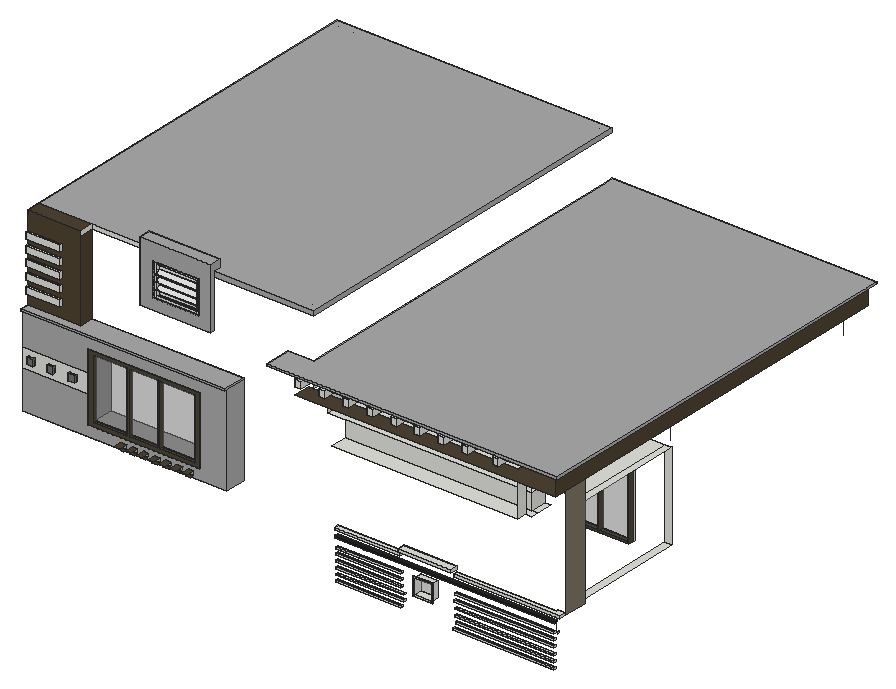
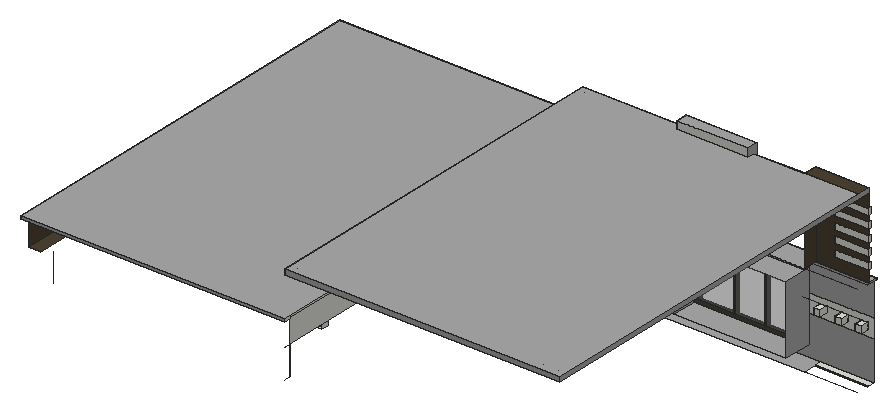
# SketchUp Ruby script. Lengths in inches.
U = 1.inch
M = Sketchup.active_model
def pt(a) = Geom::Point3d.new(a.map { |v| v * U })
def face(e, loops, mat)
  f = e.add_face(loops[0].map { |a| pt(a) })
  loops[1..].each { |l| e.add_face(l.map { |a| pt(a) }).erase! }
  f.material = f.back_material = mat if mat
  f
end
# faces: each face lists its corners as indices into pts; further lists are holes
def faces(e, pts, list, mat = nil) = list.each { |f| face(e, (f[0].is_a?(Array) ? f : [f]).map { |l| l.map { |i| pts[i] } }, mat) }
# xy, xz, yz: faces in a plane at the given z, y or x. An outline is a flat list of corners, or four numbers for a rectangle; further outlines are holes
def ring(l) = l.size == 4 ? [[l[0], l[1]], [l[2], l[1]], [l[2], l[3]], [l[0], l[3]]] : l.each_slice(2).to_a
def flat(e, list, mat, &to3) = list.each { |f| face(e, (f[0].is_a?(Array) ? f : [f]).map { |l| ring(l).map { |u, v| to3.(u, v) } }, mat) }
def xy(e, z, list, mat = nil) = flat(e, list, mat) { |x, y| [x, y, z] }
def xz(e, y, list, mat = nil) = flat(e, list, mat) { |x, z| [x, y, z] }
def yz(e, x, list, mat = nil) = flat(e, list, mat) { |y, z| [x, y, z] }
def lines(e, pts, list) = list.each { |a, b| e.add_line(pt(pts[a]), pt(pts[b])) }
# prism: a flat outline (further loops are holes) pulled along v
def prism(e, loops, v, mat = nil)
  f = face(e, loops, mat); d = Geom::Vector3d.new(v.map { |x| x * U })
  f.pushpull(f.normal.samedirection?(d) ? d.length : -d.length)
end
def box(e, o, s, mat = nil) = prism(e, [[o, [o[0] + s[0], o[1], o[2]], [o[0] + s[0], o[1] + s[1], o[2]], [o[0], o[1] + s[1], o[2]]]], [0, 0, s[2]], mat)
def at(x, y, z, deg = 0) = Geom::Transformation.translation(pt([x, y, z])) * Geom::Transformation.rotation(ORIGIN, Z_AXIS, deg.degrees)
def axes(o, x, y, z) = Geom::Transformation.new([*x, 0, *y, 0, *z, 0, *pt(o).to_a, 1])
def part(name) = M.definitions.add(name)
# library, detail: a bought-in or finely detailed component or shape, given as its bounding box
def library(name, o, s) = part(name).tap { |d| box(d.entities, o, s) }
def detail(e, o, s) = box(e.add_group.entities, o, s)
def put(e, d, t, mat = nil) = e.add_instance(d, t).tap { |i| i.material = mat if mat }
def group(e, t, mat = nil) = e.add_group.tap { |g| g.transformation = t; g.material = mat if mat }.entities
root = M.entities
M.materials.add("[Color B08]").color = [76, 71, 58]
M.materials.add("[Color C08]").color = [78, 67, 50]
M.materials.add("[Color M03]").color = [170, 170, 170]
M.materials.add("[Color M05]").color = [114, 114, 114]
M.materials.add("[Color M08]").color = [30, 30, 30]
M.materials.add("[Mirror 02]").color = [229, 229, 229]
M.materials.add("[Stone Flagstone Ashlar]1").color = [126, 116, 102]
M.materials.add("[Translucent Glass Gray]").color = [128, 128, 128]
M.materials["[Translucent Glass Gray]"].alpha = 0.5
c1 = part("Group\#2")
xy(c1.entities,0,[[0,0,90.375,3.1875]],"[Color B08]")
xy(c1.entities,4.18,[[4.18,0,31.5,3.1875],[31.5,0,33.18,3.1875],[33.18,0,56.375,3.1875],[56.375,0,58.06,3.1875],[58.06,0,86.19,3.1875]],"[Color B08]")
xy(c1.entities,71.26,[[4.18,0,31.5,3.1875],[33.18,0,56.375,3.1875],[58.06,0,86.19,3.1875]],"[Color B08]")
xy(c1.entities,75.4375,[[0,0,90.375,3.1875]],"[Color B08]")
xz(c1.entities,0,[[[0,0,90.375,75.4375],[4.18,4.18,4.18,71.26,31.5,71.26,31.5,4.18,33.18,4.18,33.18,71.26,56.375,71.26,56.375,4.18,58.06,4.18,58.06,71.26,86.19,71.26,86.19,4.18]]],"[Color B08]")
xz(c1.entities,3.1875,[[[0,0,90.375,75.4375],[4.18,4.18,86.19,4.18,86.19,71.26,58.06,71.26,58.06,4.18,56.375,4.18,56.375,71.26,33.18,71.26,33.18,4.18,31.5,4.18,31.5,71.26,4.18,71.26]]],"[Color B08]")
xz(c1.entities,3.1875,[[4.18,4.18,31.5,71.26],[33.18,4.18,56.375,71.26],[58.06,4.18,86.19,71.26]],"[Translucent Glass Gray]")
yz(c1.entities,0,[[0,0,3.1875,75.4375]],"[Color B08]")
yz(c1.entities,4.18,[[0,4.18,3.1875,71.26]],"[Color B08]")
yz(c1.entities,31.5,[[0,4.18,3.1875,71.26]],"[Color B08]")
yz(c1.entities,33.18,[[0,4.18,3.1875,71.26]],"[Color B08]")
yz(c1.entities,56.375,[[0,4.18,3.1875,71.26]],"[Color B08]")
yz(c1.entities,58.06,[[0,4.18,3.1875,71.26]],"[Color B08]")
yz(c1.entities,86.19,[[0,4.18,3.1875,71.26]],"[Color B08]")
yz(c1.entities,90.375,[[0,0,3.1875,75.4375]],"[Color B08]")
box(root,[394.1875,137.57,204.05],[82.8125,1.69,1.43])
box(root,[395.9375,137.57,209.3],[81.0625,1.69,1.43])
box(root,[297.76,137.5,210.54],[56,1.68,1.43])
box(root,[395.5625,137.57,214.55],[81.4375,1.69,1.43])
box(root,[297.76,137.5,215.47],[55.93,1.68,1.44])
box(root,[395.4375,137.57,219.8],[81.5625,1.69,1.43])
box(root,[395.0625,137.57,225.05],[81.9375,1.69,1.43])
xy(root,205.6,[[297.76,137.5,351.41,139.18]])
xy(root,207.04,[[297.76,137.5,351.41,139.18]])
xy(root,220.41,[[297.76,137.5,351.41,139.18]])
xy(root,220.77,[[364.68,133.4375,380.63,134]])
xy(root,221.65,[[365.56,133.4375,379.75,140]])
xy(root,221.85,[[297.76,137.5,351.41,139.18]])
xy(root,225.35,[[297.76,137.5,351.41,139.18]])
xy(root,226.79,[[297.76,137.5,351.41,139.18]])
xy(root,230.29,[[297.76,137.5,351.41,139.18]])
xy(root,230.3,[[395.45,137.57,477,139.26]])
xy(root,231.72,[[297.76,137.5,351.41,139.18]])
xy(root,231.73,[[395.45,137.57,477,139.26]])
xy(root,234.53,[[365.56,133.4375,379.75,140]])
xy(root,235.41,[[364.68,133.4375,380.63,134]])
xy(root,236.42,[[398.45,250.9375,448.01,256.9375]])
xy(root,238.64,[[321.84,136.1875,324.02,136.85],[436.79,136.1875,439.16,136.85],[297.76,136.85,321.84,139.48],[321.84,136.85,324.02,139.48],[324.02,136.85,436.79,139.48],
  [436.79,136.85,439.16,139.48],[439.16,136.85,477.88,139.48],[321.84,139.48,324.02,140],[436.79,139.48,439.16,140]],"[Color M08]")
xy(root,240.27,[[297.76,136.85,477.88,139.48]],"[Color M08]")
xy(root,244.375,[[297.76,136.1875,351.41,140],[395.45,136.1875,477,140],[477,136.1875,483,141.8125]])
xy(root,246.375,[[297.76,136.1875,351.41,140],[395.45,136.1875,483,136.1875,483,141.8125,477,141.8125,477,140,395.45,140]])
xy(root,248,[[351.41,134,395.45,140],[477,161.5,483,250.9375]])
xy(root,250.4375,[[351.41,134,395.45,140]])
xy(root,255.68,[[57,117.0625,100.7,122.5625],[57,122.5625,100.7,123.75]])
xy(root,255.68,[[100.7,117.0625,224.8125,134]],"[Color M03]")
xy(root,257.55,[[138.22,113.92,142.66,117.0625],[147.41,113.92,151.85,117.0625],[156.6,113.92,161.03,117.0625],[165.78,113.92,170.22,117.0625],[174.97,113.92,179.41,117.0625],
  [184.16,113.92,188.6,117.0625],[193.35,113.92,197.78,117.0625]],"[Color C08]")
xy(root,261.3,[[138.22,109.625,142.66,117.0625],[147.41,109.625,151.85,117.0625],[156.6,109.625,161.03,117.0625],[165.78,109.625,170.22,117.0625],[174.97,109.625,179.41,117.0625],
  [184.16,109.625,188.6,117.0625],[193.35,109.625,197.78,117.0625]],"[Color C08]")
xy(root,264.625,[[110.92,117.0625,202.92,140]],"[Color M03]")
xy(root,284,[[310.04,250.9375,358.04,256.9375]])
xy(root,291.17,[[398.45,250.9375,448.01,256.9375]])
xy(root,292.91,[[61.94,117.0625,67.26,123.75],[78.26,117.0625,83.57,123.75],[96.13,117.0625,101.44,123.75]])
xy(root,292.91,[[61.94,115.0625,67.26,117.0625],[78.26,115.0625,83.57,117.0625],[96.13,115.0625,101.44,117.0625]],"[Color M05]")
xy(root,298.22,[[61.94,117.0625,67.26,123.75],[78.26,117.0625,83.57,123.75],[96.13,117.0625,101.44,123.75]])
xy(root,298.22,[[61.94,115.0625,67.26,117.0625],[78.26,115.0625,83.57,117.0625],[96.13,115.0625,101.44,117.0625]],"[Color M05]")
xy(root,307.0625,[[297.76,134,297.76,148.25,455.38,148.25,455.38,141.8125,450.07,141.8125,450.07,134],[450.07,148.25,455.38,161.5]])
xy(root,320,[[282.75,148.25,282.75,250.9375,477,250.9375,477,161.5,450.07,161.5,450.07,148.25],[477,161.5,483,250.9375]])
xy(root,320.75,[[110.92,117.0625,202.92,140]],"[Color M03]")
xy(root,330.3,[[57,114.8125,224.8125,117.0625]],"[Color M03]")
xy(root,331.68,[[57,114.8125,224.8125,114.8125,224.8125,134,100.7,134,100.7,122.5625,57,122.5625]],"[Color M03]")
xy(root,340.7,[[57,120.3125,85,122.5625]])
xy(root,344,[[278.5625,119.875,278.5625,134,450.07,134,450.07,141.8125,483,141.8125,483,440,492.4375,440,492.4375,119.875]],"[Color C08]")
xy(root,345.82,[[57,120.3125,85,122.5625]])
xy(root,350.76,[[57,120.3125,85,122.5625]])
xy(root,355.88,[[57,120.3125,85,122.5625]])
xy(root,356.93,[[286.08,110.5,290.89,119.875],[305.64,110.5,310.46,119.875],[325.21,110.5,330.02,119.875],[344.77,110.5,349.58,119.875],[364.33,110.5,369.14,119.875],
  [383.89,110.5,388.71,119.875],[403.46,110.5,408.27,119.875],[423.02,110.5,427.83,119.875],[447.96,110.5,452.77,119.875]])
xy(root,358,[[142.38,130.5,200.45,134]],"[Color M03]")
xy(root,360.82,[[57,120.3125,85,122.5625]])
xy(root,362.625,[[286.08,110.5,290.89,112.3125],[305.64,110.5,310.46,112.3125],[325.21,110.5,330.02,112.3125],[344.77,110.5,349.58,112.3125],[364.33,110.5,369.14,112.3125],
  [383.89,110.5,388.71,112.3125],[403.46,110.5,408.27,112.3125],[423.02,110.5,427.83,112.3125],[447.96,110.5,452.77,112.3125],[264.5625,119.875,264.5625,134,282.75,134,282.75,256.9375,283.22,434,282.75,434,282.75,440,492.4375,440,492.4375,119.875]])
xy(root,362.625,[[261.625,112.3125,261.625,134,264.5625,134,264.5625,119.875,286.08,119.875,286.08,112.3125],[290.89,112.3125,305.64,119.875],[310.46,112.3125,325.21,119.875],[330.02,112.3125,344.77,119.875],[349.58,112.3125,364.33,119.875],
  [369.14,112.3125,383.89,119.875],[388.71,112.3125,403.46,119.875],[408.27,112.3125,423.02,119.875],[427.83,112.3125,447.96,119.875],[452.77,112.3125,452.77,119.875,492.4375,119.875,492.4375,440,499.5625,440,499.5625,112.3125]],"[Color M03]")
xy(root,364.625,[[261.625,112.3125,499.5625,112.3125,499.5625,440,282.75,440,282.75,434,283.22,434,282.75,256.9375,282.75,134,261.625,134]],"[Color M03]")
xy(root,365.95,[[57,120.3125,85,122.5625]])
xy(root,367.19,[[153.29,130.5,191.16,140]],"[Color M03]")
xy(root,370.88,[[57,120.3125,85,122.5625]])
xy(root,376.01,[[57,120.3125,85,122.5625]])
xy(root,380.95,[[57,120.3125,85,122.5625]])
xy(root,386.07,[[57,120.3125,85,122.5625]])
xy(root,394.44,[[153.29,130.5,191.16,140]],"[Color M03]")
xy(root,401.5625,[[57,122.5625,100.7,134]],"[Color C08]")
xy(root,401.5625,[[57,134,142.38,134,142.38,140,200.45,140,200.45,134,282.75,134,282.75,440,57,440]],"[Color M03]")
xy(root,408.0625,[[142.38,130.5,200.45,140]],"[Color M03]")
xz(root,110.5,[[286.08,356.93,290.89,362.625],[305.64,356.93,310.46,362.625],[325.21,356.93,330.02,362.625],[344.77,356.93,349.58,362.625],[364.33,356.93,369.14,362.625],
  [383.89,356.93,388.71,362.625],[403.46,356.93,408.27,362.625],[423.02,356.93,427.83,362.625],[447.96,356.93,452.77,362.625]])
xz(root,112.3125,[[261.625,362.625,499.5625,364.625]],"[Color M03]")
xz(root,114.8125,[[57,330.3,224.8125,331.68]],"[Color M03]")
xz(root,115.0625,[[61.94,292.91,67.26,298.22],[78.26,292.91,83.57,298.22],[96.13,292.91,101.44,298.22]],"[Color M05]")
xz(root,117.0625,[[[57,287.69,110.92,302.97],[61.94,292.91,67.26,298.22],[78.26,292.91,83.57,298.22],[96.13,292.91,101.44,298.22]]])
xz(root,117.0625,[[[57,255.68,224.8125,255.68,224.8125,330.3,57,330.3,57,302.97,110.92,302.97,110.92,320.75,202.92,320.75,202.92,264.625,110.92,264.625,110.92,287.69,57,287.69],[138.22,257.55,142.66,261.3],[147.41,257.55,151.85,261.3],[156.6,257.55,161.03,261.3],[165.78,257.55,170.22,261.3],[174.97,257.55,179.41,261.3],[184.16,257.55,188.6,261.3],[193.35,257.55,197.78,261.3]],[138.22,257.55,142.66,261.3],[147.41,257.55,151.85,261.3],[156.6,257.55,161.03,261.3],[165.78,257.55,170.22,261.3],
  [174.97,257.55,179.41,261.3],[184.16,257.55,188.6,261.3],[193.35,257.55,197.78,261.3]],"[Color M03]")
xz(root,117.0625,[[61.94,292.91,67.26,298.22],[78.26,292.91,83.57,298.22],[96.13,292.91,101.44,298.22]],"[Color M05]")
xz(root,119.875,[[286.08,356.93,290.89,362.625],[305.64,356.93,310.46,362.625],[325.21,356.93,330.02,362.625],[344.77,356.93,349.58,362.625],[364.33,356.93,369.14,362.625],
  [383.89,356.93,388.71,362.625],[403.46,356.93,408.27,362.625],[423.02,356.93,427.83,362.625],[447.96,356.93,452.77,362.625]])
xz(root,120.3125,[[57,340.7,85,345.82],[57,350.76,85,355.88],[57,360.82,85,365.95],[57,370.88,85,376.01],[57,380.95,85,386.07]])
xz(root,122.5625,[[57,340.7,85,345.82],[57,350.76,85,355.88],[57,360.82,85,365.95],[57,370.88,85,376.01],[57,380.95,85,386.07]])
xz(root,122.5625,[[57,331.68,100.7,331.68,100.7,401.5625,57,401.5625,57,386.07,85,386.07,85,380.95,57,380.95,57,376.01,85,376.01,85,370.88,57,370.88,57,365.95,85,365.95,85,360.82,57,360.82,57,355.88,85,355.88,85,350.76,57,350.76,57,345.82,85,345.82,85,340.7,57,340.7]],"[Color C08]")
xz(root,123.75,[[61.94,292.91,67.26,298.22],[78.26,292.91,83.57,298.22],[96.13,292.91,101.44,298.22]])
xz(root,130.5,[[[142.38,358,200.45,408.0625],[153.29,367.19,191.16,394.44]]],"[Color M03]")
xz(root,133.4375,[[[364.68,220.77,380.63,235.41],[365.56,221.65,379.75,234.53]]])
xz(root,134,[[351.41,248,395.45,250.4375],[100.7,330.3,224.8125,331.68],[261.625,362.625,282.75,364.625],[100.7,397.5625,142.38,401.5625]])
xz(root,134,[[200.45,397.5625,282.75,401.5625]],"[Color M03]")
xz(root,136.1875,[[297.76,244.375,351.41,246.375],[395.45,244.375,483,246.375]])
xz(root,136.85,[[297.76,238.64,477.88,240.27]],"[Color M08]")
xz(root,137.5,[[297.76,205.6,351.41,207.04],[297.76,220.41,351.41,221.85],[297.76,225.35,351.41,226.79],[297.76,230.29,351.41,231.72]])
xz(root,137.57,[[395.45,230.3,477,231.73]])
xz(root,139.18,[[297.76,205.6,351.41,207.04],[297.76,220.41,351.41,221.85],[297.76,225.35,351.41,226.79],[297.76,230.29,351.41,231.72]])
xz(root,139.26,[[395.45,230.3,477,231.73]])
xz(root,139.48,[[297.76,238.64,477.88,240.27]],"[Color M08]")
xz(root,140,[[297.76,244.375,351.41,246.375],[395.45,244.375,477,246.375],[351.41,248,395.45,250.4375],[142.38,401.5625,200.45,408.0625]])
xz(root,140,[[365.56,221.65,379.75,234.53]],"[Translucent Glass Gray]")
xz(root,141.8125,[[477,244.375,483,246.375]])
xz(root,148.25,[[297.76,307.0625,450.07,320]])
xz(root,250.9375,[[477,248,483,320],[282.75,320,282.75,344,276.75,344]])
xz(root,434,[[282.75,320,283.22,344],[282.75,344,283.22,362.625],[282.75,362.625,283.22,364.625]])
xz(root,440,[[282.75,362.625,499.5625,364.625],[57,397.5625,282.75,401.5625]],"[Color M03]")
yz(root,57,[[120.3125,340.7,122.5625,345.82],[120.3125,350.76,122.5625,355.88],[120.3125,360.82,122.5625,365.95],[120.3125,370.88,122.5625,376.01],[120.3125,380.95,122.5625,386.07]])
yz(root,57,[[114.8125,330.3,122.5625,331.68],[122.5625,397.5625,440,401.5625]],"[Color M03]")
yz(root,61.94,[[117.0625,292.91,123.75,298.22]])
yz(root,61.94,[[115.0625,292.91,117.0625,298.22]],"[Color M05]")
yz(root,67.26,[[117.0625,292.91,123.75,298.22]])
yz(root,67.26,[[115.0625,292.91,117.0625,298.22]],"[Color M05]")
yz(root,78.26,[[117.0625,292.91,123.75,298.22]])
yz(root,78.26,[[115.0625,292.91,117.0625,298.22]],"[Color M05]")
yz(root,83.57,[[117.0625,292.91,123.75,298.22]])
yz(root,83.57,[[115.0625,292.91,117.0625,298.22]],"[Color M05]")
yz(root,85,[[120.3125,340.7,122.5625,345.82],[120.3125,350.76,122.5625,355.88],[120.3125,360.82,122.5625,365.95],[120.3125,370.88,122.5625,376.01],[120.3125,380.95,122.5625,386.07]])
yz(root,96.13,[[117.0625,292.91,123.75,298.22]])
yz(root,96.13,[[115.0625,292.91,117.0625,298.22]],"[Color M05]")
yz(root,100.7,[[122.5625,397.5625,134,401.5625]])
yz(root,100.7,[[122.5625,331.68,134,397.5625]],"[Color C08]")
yz(root,101.44,[[117.0625,292.91,123.75,298.22]])
yz(root,101.44,[[115.0625,292.91,117.0625,298.22]],"[Color M05]")
yz(root,110.92,[[117.0625,264.625,140,320.75]],"[Color M03]")
yz(root,142.38,[[130.5,358,130.5,408.0625,140,408.0625,140,401.5625,134,401.5625,134,358]],"[Color M03]")
yz(root,153.29,[[130.5,367.19,140,394.44]],"[Color M03]")
yz(root,191.16,[[130.5,367.19,140,394.44]],"[Color M03]")
yz(root,200.45,[[130.5,358,134,358,134,401.5625,140,401.5625,140,408.0625,130.5,408.0625]],"[Color M03]")
yz(root,202.92,[[117.0625,264.625,140,320.75]],"[Color M03]")
yz(root,224.8125,[[117.0625,255.68,134,330.3],[114.8125,330.3,134,331.68]],"[Color M03]")
yz(root,261.625,[[112.3125,362.625,134,364.625]],"[Color M03]")
yz(root,282.75,[[148.25,320,250.9375,344],[250.9375,320,256.9375,344],[134,344,140,362.625],[140,344,148.25,362.625],[148.25,344,250.9375,362.625],
  [250.9375,344,256.9375,362.625],[134,362.625,140,364.625],[140,362.625,148.25,364.625],[148.25,362.625,250.9375,364.625],[250.9375,362.625,256.9375,364.625],
  [434,362.625,440,364.625]])
yz(root,282.75,[[134,397.5625,440,401.5625]],"[Color M03]")
yz(root,286.08,[[110.5,356.93,119.875,362.625]])
yz(root,290.89,[[110.5,356.93,119.875,362.625]])
yz(root,297.76,[[137.5,205.6,139.18,207.04],[137.5,220.41,139.18,221.85],[137.5,225.35,139.18,226.79],[137.5,230.29,139.18,231.72],[136.1875,244.375,140,246.375]])
yz(root,297.76,[[136.85,238.64,139.48,240.27]],"[Color M08]")
yz(root,305.64,[[110.5,356.93,119.875,362.625]])
yz(root,310.46,[[110.5,356.93,119.875,362.625]])
yz(root,325.21,[[110.5,356.93,119.875,362.625]])
yz(root,330.02,[[110.5,356.93,119.875,362.625]])
yz(root,344.77,[[110.5,356.93,119.875,362.625]])
yz(root,349.58,[[110.5,356.93,119.875,362.625]])
yz(root,351.41,[[136.1875,244.375,140,246.375],[136.1875,246.375,140,248],[134,248,136.1875,250.4375],[136.1875,248,140,250.4375]])
yz(root,364.33,[[110.5,356.93,119.875,362.625]])
yz(root,364.68,[[133.4375,220.77,134,235.41]])
yz(root,365.56,[[133.4375,221.65,140,234.53]])
yz(root,369.14,[[110.5,356.93,119.875,362.625]])
yz(root,379.75,[[133.4375,221.65,140,234.53]])
yz(root,380.63,[[133.4375,220.77,134,235.41]])
yz(root,383.89,[[110.5,356.93,119.875,362.625]])
yz(root,388.71,[[110.5,356.93,119.875,362.625]])
yz(root,395.45,[[136.1875,244.375,140,246.375],[134,248,140,250.4375]])
yz(root,398.45,[[250.9375,236.42,256.9375,291.17]])
yz(root,403.46,[[110.5,356.93,119.875,362.625]])
yz(root,408.27,[[110.5,356.93,119.875,362.625]])
yz(root,423.02,[[110.5,356.93,119.875,362.625]])
yz(root,427.83,[[110.5,356.93,119.875,362.625]])
yz(root,447.96,[[110.5,356.93,119.875,362.625]])
yz(root,448.01,[[250.9375,236.42,256.9375,291.17]])
yz(root,450.07,[[134,307.0625,141.8125,344],[148.25,307.0625,161.5,320]])
yz(root,452.77,[[110.5,356.93,119.875,362.625]])
yz(root,477,[[137.57,230.3,139.26,231.73],[140,244.375,141.8125,246.375]])
yz(root,477.88,[[136.85,238.64,139.48,240.27]],"[Color M08]")
yz(root,478.5625,[[139.18,230.29,140,231.72],[140,230.29,140.87,231.72]])
yz(root,483,[[136.1875,244.375,141.8125,246.375]])
yz(root,483,[[141.8125,244.375,161.5,344]],"[Stone Flagstone Ashlar]1")
yz(root,492.4375,[[119.875,344,440,362.625]],"[Color C08]")
yz(root,499.5625,[[112.3125,362.625,440,364.625]],"[Color M03]")
p = [[283.22,434,344],[282.75,256.9375,344],[282.75,256.9375,362.625],[283.22,434,362.625],[282.75,256.9375,364.625],[283.22,434,364.625],
  [282.75,434,320],[282.75,440,320],[477,434,320],[477,434,344],[477,256.9375,320],[477,256.9375,344],
  [450.07,148.25,320],[450.07,148.25,344],[282.75,434,344],[282.75,440,344],[63,140,397.5625],[276.75,140,397.5625],
  [57,134,255.68],[100.7,134,255.68],[100.7,134,331.68],[57,134,331.68],[110.92,123.75,302.97],[57,123.75,302.97],
  [224.8125,123.75,330.3],[57,123.75,330.3],[477,140,244.375],[477,140,231.72],[74.8,434,397.5625],[74.8,434,401.5625],
  [63,434,397.5625],[63,434,401.5625],[276.75,140,401.5625],[276.75,434,397.5625],[276.75,434,401.5625]]
faces(root,p,[[0,1,2,3],[3,2,4,5]])
lines(root,p,[[6,7],[8,9],[10,11],[12,13],[14,15],[16,17],[18,19],[20,21],[22,23],[24,25],[26,27],[28,29],
  [30,31],[17,32],[33,34]])
g1 = group(root,at(398.45,250.9375,236.42))
xy(g1,0,[[0,0,49.5625,4.14]],"[Color B08]")
xy(g1,1.25,[[1.14,0,23.57,4.14],[23.57,0,24.78,4.14],[24.78,0,48.43,4.14]],"[Color B08]")
xy(g1,53.51,[[1.14,0,23.57,4.14],[24.78,0,48.43,4.14]],"[Color B08]")
xy(g1,54.76,[[0,0,49.5625,4.14]],"[Color B08]")
xz(g1,0,[[[0,0,49.5625,54.76],[1.14,1.25,1.14,53.51,23.57,53.51,23.57,1.25,24.78,1.25,24.78,53.51,48.43,53.51,48.43,1.25]]],"[Color B08]")
xz(g1,4.14,[[[0,0,49.5625,54.76],[1.14,1.25,48.43,1.25,48.43,53.51,24.78,53.51,24.78,1.25,23.57,1.25,23.57,53.51,1.14,53.51]]],"[Color B08]")
xz(g1,4.14,[[1.14,1.25,23.57,53.51],[24.78,1.25,48.43,53.51]],"[Translucent Glass Gray]")
yz(g1,0,[[0,0,4.14,54.76]],"[Color B08]")
yz(g1,1.14,[[0,1.25,4.14,53.51]],"[Color B08]")
yz(g1,23.57,[[0,1.25,4.14,53.51]],"[Color B08]")
yz(g1,24.78,[[0,1.25,4.14,53.51]],"[Color B08]")
yz(g1,48.43,[[0,1.25,4.14,53.51]],"[Color B08]")
yz(g1,49.5625,[[0,0,4.14,54.76]],"[Color B08]")
put(root,c1,axes([110.92,117.0625,264.625],[1.01798,0,0],[0,0.81996,0],[0,0,0.74399]))
g2 = group(root,at(153.29,130.57,367.19))
xy(g2,0,[[0,0.41,37.875,2.614]])
xy(g2,1.854,[[2.577,0.41,35.298,2.614]])
xy(g2,13.223,[[2.562,0.41,2.567,2.614]])
xy(g2,15.2,[[2.562,0.41,2.565,2.614]])
xy(g2,25.396,[[2.577,0.41,35.298,2.614]])
xy(g2,27.25,[[0,0.41,37.875,2.614]])
xz(g2,0,[[2.572,6.189,35.284,6.189,35.284,6.59,2.57,6.59],[2.562,17.805,35.284,18.004]])
xz(g2,0,[[2.567,12.116,35.284,12.116,35.284,12.455,2.565,12.455]],"[Mirror 02]")
xz(g2,0.41,[[[0,0,37.875,27.25],[2.577,1.854,2.572,6.403,2.57,9.53,2.567,12.289,2.567,13.223,2.562,13.223,2.562,15.2,2.565,15.2,2.5625,18.003,2.562,18.481,2.562,21.044,2.577,25.396,35.298,25.396,35.284,21.044,35.284,18.003,35.298,1.854]]])
xz(g2,2.614,[[[0,0,37.875,27.25],[2.577,1.854,35.298,1.854,35.284,19.066,35.284,21.044,35.298,25.396,2.577,25.396,2.562,21.044,2.562,19.066,2.565,15.2,2.562,15.2,2.562,13.223,2.567,13.223,2.57,9.53,2.572,7.553],[2.562,7.553,35.284,9.53]],[2.562,7.553,2.562,9.53,2.565,9.53,2.567,7.553],[2.567,7.553,2.572,7.553,2.57,9.53,2.565,9.53],[2.562,13.223,2.567,13.223,2.565,15.2,2.562,15.2]])
xz(g2,2.614,[[2.577,1.854,35.298,1.854,35.284,19.066,2.562,19.066,2.565,15.2,35.284,15.2,35.284,13.223,2.567,13.223,2.57,9.53,35.284,9.53,35.284,7.553,2.572,7.553],[2.572,7.553,2.57,9.53,35.284,9.53,35.284,7.553],[2.567,13.223,2.565,15.2,35.284,15.2,35.284,13.223],[2.562,19.066,35.284,21.044],[2.562,21.044,35.284,21.044,35.298,25.396,2.577,25.396]],"[Mirror 02]")
yz(g2,0,[[0.41,0,2.614,27.25]])
yz(g2,2.562,[[0.41,13.223,2.614,15.2],[0.41,19.066,0.913,19.066,2.614,21.044,0.41,21.044],[0.913,19.066,2.614,21.044,2.614,19.066]])
yz(g2,35.284,[[0,6.189,2.614,7.553,0.856,7.553,0,6.59],[0.856,7.553,2.614,7.553,2.614,9.53],[0,12.116,2.614,13.223,2.614,15.2,0,12.455],[0,17.805,0.41,18.003,0.41,18.481,0,18.004],[0.41,18.003,2.614,19.066,0.913,19.066,0.41,18.481],
  [0.41,19.066,0.41,21.044,2.614,21.044,0.913,19.066],[0.913,19.066,2.614,19.066,2.614,21.044]])
yz(g2,37.875,[[0.41,0,2.614,27.25]])
p = [[2.577,2.614,1.854],[2.572,2.614,7.553],[2.57,2.614,9.53],[2.567,2.614,13.223],[2.567,0.41,13.223],[2.567,0.41,12.289],
  [2.57,0.41,9.53],[2.572,0.41,6.403],[2.577,0.41,1.854],[35.284,2.614,19.066],[35.298,2.614,1.854],[35.298,0.41,1.854],
  [35.284,0.41,18.003],[35.284,0.41,18.481],[35.284,0.41,19.066],[35.284,0.913,19.066],[35.284,2.614,7.553],[35.284,0,6.189],
  [2.572,0,6.189],[2.57,0,6.59],[35.284,0,6.59],[35.284,0.856,7.553],[35.284,2.614,9.53],[2.567,0,12.116],
  [2.565,0,12.455],[35.284,2.614,13.223],[35.284,0,12.116],[35.284,0,12.455],[35.284,2.614,15.2],[2.565,2.614,15.2],
  [2.562,2.614,19.066],[2.562,0.913,19.066],[2.562,0.41,19.066],[2.562,0.41,18.481],[2.5625,0.41,18.003],[2.565,0.41,15.2],
  [2.562,0,18.004],[2.562,0,17.805],[35.284,0,17.805],[35.284,0,18.004],[35.284,2.614,21.044],[2.562,2.614,21.044],
  [2.577,2.614,25.396],[2.577,0.41,25.396],[2.562,0.41,21.044],[35.298,2.614,25.396],[35.284,0.41,21.044],[35.298,0.41,25.396],
  [2.565,0.41,9.53]]
faces(g2,p,[[0,1,2,3,4,5,6,7,8],[9,10,11,12,13,14,15],[1,16,17,18,7],[18,19,1,7],[2,1,19],[23,24,3,5],[3,25,26,23,5],[29,3,24],
  [29,30,31,32,33,34,35],[36,33,34,37],[30,9,12,38,37,34],[33,31,30,34],[41,42,43,44],[45,40,46,47]])
faces(g2,p,[[19,20,21,22,2],[24,27,28,29],[36,39,13,15,40,41,31,33]],"[Mirror 02]")
lines(g2,p,[[6,48]])
